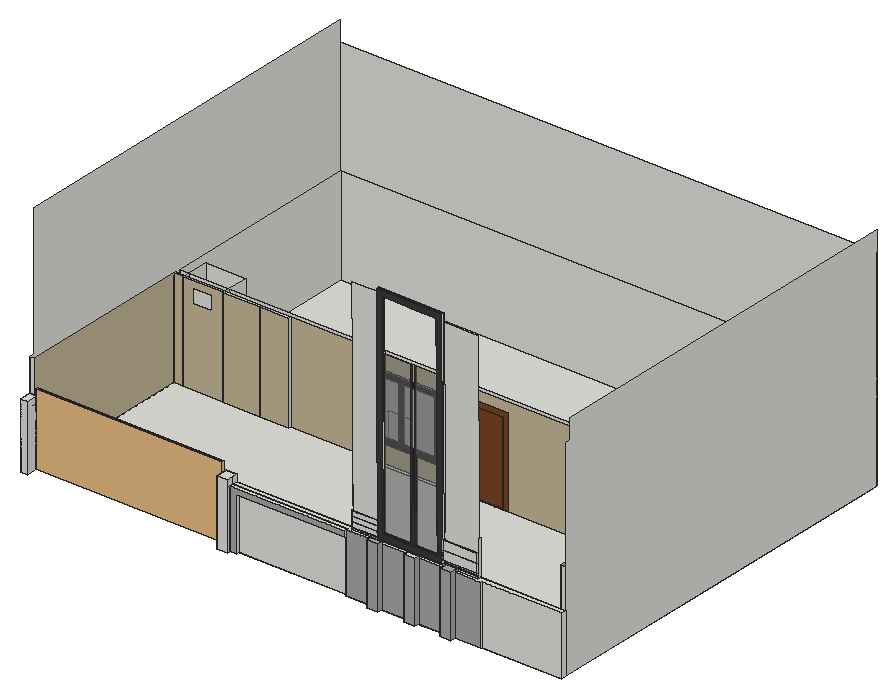
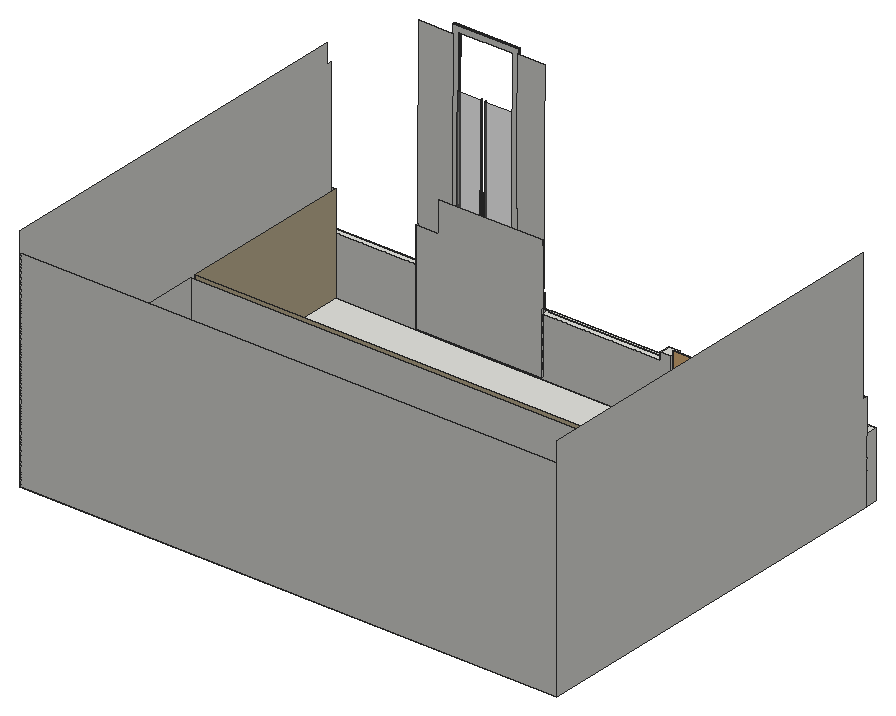
# SketchUp Ruby script. Lengths in inches.
U = 1.inch
M = Sketchup.active_model
def pt(a) = Geom::Point3d.new(a.map { |v| v * U })
def face(e, loops, mat)
  f = e.add_face(loops[0].map { |a| pt(a) })
  loops[1..].each { |l| e.add_face(l.map { |a| pt(a) }).erase! }
  f.material = f.back_material = mat if mat
  f
end
# faces: each face lists its corners as indices into pts; further lists are holes
def faces(e, pts, list, mat = nil) = list.each { |f| face(e, (f[0].is_a?(Array) ? f : [f]).map { |l| l.map { |i| pts[i] } }, mat) }
# xy, xz, yz: faces in a plane at the given z, y or x. An outline is a flat list of corners, or four numbers for a rectangle; further outlines are holes
def ring(l) = l.size == 4 ? [[l[0], l[1]], [l[2], l[1]], [l[2], l[3]], [l[0], l[3]]] : l.each_slice(2).to_a
def flat(e, list, mat, &to3) = list.each { |f| face(e, (f[0].is_a?(Array) ? f : [f]).map { |l| ring(l).map { |u, v| to3.(u, v) } }, mat) }
def xy(e, z, list, mat = nil) = flat(e, list, mat) { |x, y| [x, y, z] }
def xz(e, y, list, mat = nil) = flat(e, list, mat) { |x, z| [x, y, z] }
def yz(e, x, list, mat = nil) = flat(e, list, mat) { |y, z| [x, y, z] }
def lines(e, pts, list) = list.each { |a, b| e.add_line(pt(pts[a]), pt(pts[b])) }
# prism: a flat outline (further loops are holes) pulled along v
def prism(e, loops, v, mat = nil)
  f = face(e, loops, mat); d = Geom::Vector3d.new(v.map { |x| x * U })
  f.pushpull(f.normal.samedirection?(d) ? d.length : -d.length)
end
def box(e, o, s, mat = nil) = prism(e, [[o, [o[0] + s[0], o[1], o[2]], [o[0] + s[0], o[1] + s[1], o[2]], [o[0], o[1] + s[1], o[2]]]], [0, 0, s[2]], mat)
def at(x, y, z, deg = 0) = Geom::Transformation.translation(pt([x, y, z])) * Geom::Transformation.rotation(ORIGIN, Z_AXIS, deg.degrees)
def axes(o, x, y, z) = Geom::Transformation.new([*x, 0, *y, 0, *z, 0, *pt(o).to_a, 1])
def part(name) = M.definitions.add(name)
# library, detail: a bought-in or finely detailed component or shape, given as its bounding box
def library(name, o, s) = part(name).tap { |d| box(d.entities, o, s) }
def detail(e, o, s) = box(e.add_group.entities, o, s)
def put(e, d, t, mat = nil) = e.add_instance(d, t).tap { |i| i.material = mat if mat }
def group(e, t, mat = nil) = e.add_group.tap { |g| g.transformation = t; g.material = mat if mat }.entities
root = M.entities
M.materials.add("[0132_LightGray]").color = [169, 169, 169]
M.materials.add("[Color M07]").color = [58, 58, 58]
M.materials.add("[Color M08]").color = [30, 30, 30]
M.materials.add("[Quartz Light Brown]").color = [199, 184, 152]
M.materials.add("[Translucent Glass Gray]").color = [128, 128, 128]
M.materials["[Translucent Glass Gray]"].alpha = 0.5
M.materials.add("[Wood Veneer 01]").color = [120, 70, 37]
c1 = library("gate (1)",[0,0,0],[171.26,1.97,78.74])
prism(root,[[[595.0625,24.87,16.39],[825.84,24.87,16.39],[825.84,21.87,16.375],[595.0625,21.87,16.375]]],[0,-0.1,15.6875])
prism(root,[[[595.0625,24.87,36.02],[825.84,24.87,36.02],[825.84,21.74,36],[595.0625,21.74,36]]],[0,-0.1,15.6875])
prism(root,[[[595.0625,24.87,55.64],[825.84,24.87,55.64],[825.84,21.61,55.62],[595.0625,21.61,55.62]]],[0,-0.1,15.6875])
prism(root,[[[595.0625,24.87,75.27],[825.84,24.87,75.27],[825.84,21.48,75.25],[595.0625,21.48,75.25]]],[0,-0.1,15.6875])
xy(root,0,[[0,6,13.1875,18],[360,6,379.36,18],[634.43,6,654.87,15],[702.3,6,720,15],[720,6,722.74,15],
  [768.43,6,768.43,15,720,15,720,27,982.625,27,982.625,18,836.43,18,836.43,15,788.87,15,788.87,6],[379.36,12,391.35,18],[589.74,15,589.74,18,360,18,360,27,720,27,720,15],[0,18,13.1875,27],[0,27,0,738,982.625,738,982.625,729,9,729,9,359.125,25.58,359.125,25.58,350.125,9,350.125,9,27],
  [9,27,972.875,27,972.875,350.125,220.94,350.125,220.94,345.8125,99.55,345.8125,99.55,346.125,25.58,346.125,25.58,347.125,9,347.125],[972.875,27,972.875,350.125,608.23,350.125,608.23,353.125,514.29,353.125,514.29,350.125,439.49,350.125,439.49,352.625,397.49,352.625,397.49,350.125,99.55,350.125,99.55,359.125,982.625,359.125,982.625,27],[99.55,345.8125,167.26,350.125],[167.26,345.8125,220.94,350.125],[25.58,346.125,99.55,350.125],
  [9,347.125,25.58,350.125],[25.58,350.125,99.55,359.125],[397.49,350.125,400.49,352.625],[400.49,350.125,436.49,352.625],[436.49,350.125,439.49,352.625],
  [514.29,350.125,608.23,353.125],[9,359.125,25.58,359.125,25.58,398.125,99.55,398.125,99.55,359.125,972.875,359.125,972.875,729,9,729],[25.58,359.125,99.55,398.125],[972.875,359.125,982.625,729]])
xy(root,34.12,[[343.29,347.125,496.31,350.125]])
xy(root,43.35,[[419.8,347.125,426.4375,350.125]])
xy(root,43.35,[[352.52,347.125,419.8,350.125],[426.4375,347.125,487.09,350.125]],"[Color M08]")
xy(root,96.82,[[391.35,12,589.74,18]])
xy(root,108,[[379.36,6,379.39,12],[379.36,12,379.39,18],[379.39,12,589.74,18],[589.74,15,768.43,15,768.43,21.27,788.61,21.27,788.87,15,836.43,15,836.43,18,982.625,18,982.625,27,379.39,27,379.39,18,589.74,18]])
xy(root,111.5625,[[702.3,6,722.74,15]])
xy(root,111.5625,[[634.43,6,654.87,15],[768.43,6,788.87,6,788.87,15,788.61,21.27,768.43,21.27]],"[0132_LightGray]")
xy(root,112.12,[[595.0625,21.24,644.47,22.14]])
xy(root,120,[[0,6,13.1875,27],[360,6,379.36,6,379.36,18,379.39,18,379.39,27,360,27]])
xy(root,138.72,[[595.0625,21.07,644.47,22.09]])
xz(root,6,[[0,0,13.1875,120],[360,0,379.36,120]])
xz(root,6,[[634.43,0,654.87,111.5625],[702.3,0,722.74,111.5625],[768.43,0,788.87,111.5625]],"[0132_LightGray]")
xz(root,12,[[379.36,0,391.35,0,391.35,96.82,589.74,96.82,589.74,108,379.36,108]],"[0132_LightGray]")
xz(root,15,[[634.43,0,654.87,108],[702.3,0,722.74,108],[634.43,108,654.87,111.5625],[702.3,108,722.74,111.5625]])
xz(root,15,[[589.74,0,634.43,108],[654.87,0,702.3,108],[722.74,0,768.43,108],[788.87,0,836.43,108]],"[0132_LightGray]")
xz(root,18,[[379.36,0,379.36,108,589.74,108,589.74,96.82,391.35,96.82,391.35,0],[391.35,0,589.74,96.82],[836.43,0,982.625,108],[379.36,108,379.39,120]])
xz(root,21.27,[[768.43,108,788.61,111.5625]])
xz(root,27,[[0,0,9,108],[9,0,13.1875,108],[360,0,360,120,379.39,120,379.39,108,720,108,720,0],[720,0,972.875,108],[972.875,0,982.625,108],
  [0,108,9,120],[9,108,13.1875,120],[972.875,108,982.625,180],[0,120,9,180]])
xz(root,345.8125,[[99.55,0,167.26,180],[167.26,0,220.94,180]],"[Quartz Light Brown]")
xz(root,346.125,[[[25.58,0,99.55,180],[44.38,142.05,78.26,168.55]]],"[Quartz Light Brown]")
xz(root,347.125,[[[343.29,34.12,496.31,152.83],[352.52,43.35,487.09,143.6]],[419.8,43.35,426.4375,143.6]],"[Color M08]")
xz(root,347.125,[[9,0,25.58,180]],"[Quartz Light Brown]")
xz(root,350.125,[[9,0,25.58,180],[25.58,0,99.55,180],[99.55,0,167.26,180],[167.26,0,220.94,180],[[343.29,34.12,496.31,152.83],[352.52,43.35,487.09,143.6]],
  [419.8,43.35,426.4375,143.6]])
xz(root,350.125,[[[220.94,0,502.5625,0,502.5625,163.72,619.95,163.72,619.95,0,972.875,0,972.875,180,220.94,180],[343.29,34.12,496.31,152.83]]],"[Quartz Light Brown]")
xz(root,350.125,[[352.52,43.35,419.8,143.6],[426.4375,43.35,487.09,143.6]],"[Translucent Glass Gray]")
xz(root,350.125,[[502.5625,0,514.29,0,514.29,151.99,608.23,151.99,608.23,0,619.95,0,619.95,163.72,502.5625,163.72],[542.09,54.84,546.17,55.38,549.97,56.95,553.23,59.46,555.73,62.72,557.3,66.52,557.84,70.59,557.3,74.67,555.73,78.47,553.23,81.73,549.97,84.23,546.17,85.81,542.09,86.34,538.01,85.81,534.22,84.23,530.95,81.73,528.45,78.47,526.88,74.67,526.34,70.59,526.88,66.52,528.45,62.72,530.95,59.46,534.22,56.95,538.01,55.38]],"[Wood Veneer 01]")
xz(root,352.625,[[397.49,0,439.49,87]])
xz(root,353.125,[[542.09,54.84,538.01,55.38,534.22,56.95,530.95,59.46,528.45,62.72,526.88,66.52,526.34,70.59,526.88,74.67,528.45,78.47,530.95,81.73,534.22,84.23,538.01,85.81,542.09,86.34,546.17,85.81,549.97,84.23,553.23,81.73,555.73,78.47,557.3,74.67,557.84,70.59,557.3,66.52,555.73,62.72,553.23,59.46,549.97,56.95,546.17,55.38]])
xz(root,353.125,[[[514.29,0,608.23,151.99],[542.09,54.84,538.01,55.38,534.22,56.95,530.95,59.46,528.45,62.72,526.88,66.52,526.34,70.59,526.88,74.67,528.45,78.47,530.95,81.73,534.22,84.23,538.01,85.81,542.09,86.34,546.17,85.81,549.97,84.23,553.23,81.73,555.73,78.47,557.3,74.67,557.84,70.59,557.3,66.52,555.73,62.72,553.23,59.46,549.97,56.95,546.17,55.38]]],"[Wood Veneer 01]")
xz(root,359.125,[[9,0,972.875,180]])
xz(root,398.125,[[25.58,0,99.55,180]])
xz(root,729,[[9,0,972.875,180]])
xz(root,738,[[0,0,982.625,384]])
yz(root,0,[[6,0,27,120],[27,0,27,180,36,180,36,420,738,420,738,0]])
yz(root,9,[[347.125,0,350.125,180],[359.125,0,729,180]])
yz(root,9,[[27,0,347.125,180]],"[Quartz Light Brown]")
yz(root,13.1875,[[6,0,27,120]])
yz(root,25.58,[[346.125,0,347.125,180],[347.125,0,350.125,180],[350.125,0,398.125,180]])
yz(root,99.55,[[345.8125,0,346.125,180],[346.125,0,350.125,180],[350.125,0,398.125,180]])
yz(root,167.26,[[345.8125,0,350.125,180]])
yz(root,220.94,[[345.8125,0,350.125,180]])
yz(root,343.29,[[347.125,34.12,350.125,152.83]],"[Color M08]")
yz(root,352.52,[[347.125,43.35,350.125,143.6]],"[Color M08]")
yz(root,360,[[6,0,27,120]])
yz(root,379.36,[[6,0,12,108],[12,0,18,108],[6,108,18,120]])
yz(root,379.39,[[18,108,27,120]])
yz(root,391.35,[[12,0,18,96.82]])
yz(root,419.8,[[347.125,43.35,350.125,143.6]],"[Color M08]")
yz(root,426.4375,[[347.125,43.35,350.125,143.6]],"[Color M08]")
yz(root,487.09,[[347.125,43.35,350.125,143.6]],"[Color M08]")
yz(root,496.31,[[347.125,34.12,350.125,152.83]],"[Color M08]")
yz(root,514.29,[[350.125,0,353.125,151.99]],"[Wood Veneer 01]")
yz(root,589.74,[[15,0,18,96.82],[12,96.82,15,108],[15,96.82,18,108]])
yz(root,595.0625,[[25.47,2.61,24.87,94.89,24.76,110.58,24.3125,180,27,180,27,227.94,28.47,2.63],[21.36,94.87,21.25,110.56,24.76,110.58,24.87,94.89],[21.24,112.12,21.19,120.34,22.09,120.35,22.14,112.12],[21.18,121.3,21.13,129.53,22.09,129.54,22.14,121.31],[21.125,130.49,21.07,138.72,22.09,138.72,22.14,130.5]])
yz(root,608.23,[[350.125,0,353.125,151.99]],"[Wood Veneer 01]")
yz(root,634.43,[[6,0,15,111.5625]],"[0132_LightGray]")
yz(root,644.47,[[21.76,111.28,21.75,112.12,22.14,112.12,24.75,112.14,24.76,111.3],[21.24,112.12,21.19,120.34,21.7,120.35,21.75,112.12],[21.75,112.12,21.7,120.35,22.09,120.35,22.14,112.12],[22.14,112.12,22.09,120.35,24.7,120.37,24.75,112.14],[21.7,120.35,21.69,121.31,22.14,121.31,24.69,121.33,24.7,120.37,22.09,120.35],
  [21.18,121.3,21.13,129.53,21.64,129.53,21.69,121.31],[21.69,121.31,21.64,129.53,22.09,129.54,22.14,121.31],[22.14,121.31,22.09,129.54,24.64,129.55,24.69,121.33],[21.64,129.53,21.63,130.49,22.14,130.5,24.63,130.51,24.64,129.55,22.09,129.54],[21.125,130.49,21.07,138.72,21.58,138.72,21.63,130.49],
  [21.63,130.49,21.58,138.72,22.09,138.72,22.14,130.5],[22.14,130.5,22.09,138.72,24.58,138.74,24.63,130.51],[21.58,138.72,21.57,139.68,22.14,139.68,24.57,139.7,24.58,138.74,22.09,138.72]])
yz(root,644.47,[[18.76,111.26,18.75,112.1,21.24,112.12,21.75,112.12,21.76,111.28],[18.75,112.1,18.7,120.33,21.19,120.34,21.24,112.12],[18.7,120.33,18.69,121.29,21.18,121.3,21.69,121.31,21.7,120.35,21.19,120.34],[18.69,121.29,18.64,129.51,21.13,129.53,21.18,121.3],[18.64,129.51,18.63,130.47,21.125,130.49,21.63,130.49,21.64,129.53,21.13,129.53],
  [18.63,130.47,18.58,138.7,21.07,138.72,21.125,130.49],[18.58,138.7,18.57,139.66,21.0625,139.68,21.57,139.68,21.58,138.72,21.07,138.72]],"[Color M07]")
yz(root,653.47,[[18.7,120.26,21.7,120.28,21.26,187.5,18.26,187.48],[21.7,120.28,24.7,120.3,24.26,187.52,22.78,187.51,21.26,187.5]],"[Color M07]")
yz(root,654.87,[[6,0,15,111.5625]],"[0132_LightGray]")
yz(root,702.3,[[6,0,15,111.5625]],"[0132_LightGray]")
yz(root,703.69,[[21.7,120.28,21.26,187.5,21.22,194.61,20.77,263.62,20.72,270.73,20.27,339.74,20.23,346.86,19.78,415.86,22.78,415.88,24.7,120.3]],"[Color M07]")
yz(root,710.84,[[21.7,120.28,24.7,120.3,22.78,415.88,19.78,415.86,20.23,346.86,20.27,339.74,20.72,270.73,20.77,263.62,21.22,194.61,21.26,187.5]],"[Color M07]")
yz(root,722.74,[[6,0,15,111.5625]],"[0132_LightGray]")
yz(root,753.91,[[18.7,120.26,18.26,187.48,21.26,187.5,21.7,120.28],[21.7,120.28,21.26,187.5,22.78,187.51,24.26,187.52,24.7,120.3]],"[Color M07]")
yz(root,762.91,[[18.76,111.26,21.76,111.28,21.72,117.24,20.16,117.23,18.72,117.23],[21.76,111.28,24.76,111.3,24.72,117.26,22.1875,117.25,21.72,117.24],[18.72,117.23,20.16,117.23,20.06,132.84,18.62,132.83],[20.16,117.23,21.72,117.24,21.62,132.85,20.06,132.84],[21.72,117.24,22.1875,117.25,22.09,132.85,21.62,132.85],
  [22.1875,117.25,24.72,117.26,24.62,132.87,22.09,132.85],[18.62,132.83,20.06,132.84,21.62,132.85,21.61,133.99,20.05,133.98,18.61,133.97],[21.62,132.85,22.09,132.85,24.62,132.87,24.61,134.01,22.1875,134,21.61,133.99],[18.61,133.97,20.05,133.98,19.95,149.59,18.51,149.58],[20.05,133.98,21.61,133.99,21.51,149.6,19.95,149.59],
  [21.61,133.99,22.1875,134,22.09,149.6,21.51,149.6],[22.1875,134,24.61,134.01,24.51,149.61,22.09,149.6]])
yz(root,768.43,[[6,0,6,111.5625,21.27,111.5625,21.27,108,15,108,15,0]],"[0132_LightGray]")
yz(root,788.87,[[6,0,15,111.5625]],"[0132_LightGray]")
yz(root,825.84,[[25.47,2.61,28.47,2.63,27.36,172.4375,24.36,172.42,24.76,110.58,24.87,94.89],[21.36,94.87,24.87,94.89,24.76,110.58,21.25,110.56],[20.16,117.23,22.1875,117.25,22.09,132.85,20.06,132.84],[20.05,133.98,22.1875,134,22.09,149.6,19.95,149.59]])
yz(root,836.43,[[15,0,18,108]])
yz(root,972.875,[[359.125,0,729,180]])
yz(root,972.875,[[27,0,350.125,180]],"[Quartz Light Brown]")
yz(root,982.625,[[18,0,27,108],[27,0,738,0,738,420,35.0625,420,35.0625,384,27,384]])
p = [[825.84,25.47,2.61],[825.84,24.87,94.89],[595.0625,24.87,94.89],[595.0625,25.47,2.61],[595.0625,28.47,2.63],[825.84,28.47,2.63],
  [595.0625,27,227.94],[784.34,27,227.94],[784.34,27.36,172.4375],[825.84,27.36,172.4375],[538.01,353.125,55.38],[542.09,353.125,54.84],
  [542.09,350.125,54.84],[538.01,350.125,55.38],[546.17,353.125,55.38],[546.17,350.125,55.38],[534.22,353.125,56.95],[534.22,350.125,56.95],
  [549.97,353.125,56.95],[549.97,350.125,56.95],[530.95,353.125,59.46],[530.95,350.125,59.46],[553.23,353.125,59.46],[553.23,350.125,59.46],
  [528.45,353.125,62.72],[528.45,350.125,62.72],[555.73,353.125,62.72],[555.73,350.125,62.72],[526.88,353.125,66.52],[526.88,350.125,66.52],
  [557.3,353.125,66.52],[557.3,350.125,66.52],[526.34,353.125,70.59],[526.34,350.125,70.59],[557.84,353.125,70.59],[557.84,350.125,70.59],
  [526.88,353.125,74.67],[526.88,350.125,74.67],[557.3,353.125,74.67],[557.3,350.125,74.67],[528.45,353.125,78.47],[528.45,350.125,78.47],
  [555.73,353.125,78.47],[555.73,350.125,78.47],[530.95,353.125,81.73],[530.95,350.125,81.73],[553.23,353.125,81.73],[553.23,350.125,81.73],
  [534.22,353.125,84.23],[534.22,350.125,84.23],[549.97,353.125,84.23],[549.97,350.125,84.23],[538.01,353.125,85.81],[538.01,350.125,85.81],
  [546.17,353.125,85.81],[546.17,350.125,85.81],[542.09,353.125,86.34],[542.09,350.125,86.34],[595.0625,21.25,110.56],[595.0625,21.36,94.87],
  [825.84,21.36,94.87],[825.84,21.25,110.56],[595.0625,24.76,110.58],[825.84,24.76,110.58],[788.87,15,108],[788.61,21.27,108],
  [788.61,21.27,111.5625],[788.87,15,111.5625],[595.0625,24.3125,180],[825.84,24.36,172.42],[825.84,24.28,184.45],[825.84,24.18,200.05],
  [825.84,24,227.98],[825.84,22.1875,506.25],[762.91,22.1875,506.25],[762.91,23.52,301.67],[762.91,23.62,286.07],[762.91,23.63,284.73],
  [762.91,23.73,269.13],[762.91,23.74,267.8],[762.91,23.84,252.2],[762.91,23.85,250.86],[762.91,23.95,235.26],[762.91,23.96,233.92],
  [762.91,24.0625,218.32],[762.91,24.07,216.99],[762.91,24.17,201.39],[762.91,24.18,200.05],[762.91,24.28,184.45],[762.91,24.29,183.11],
  [762.91,24.39,167.51],[762.91,24.4,166.36],[762.91,24.5,150.76],[762.91,24.51,149.61],[762.91,24.61,134.01],[762.91,24.62,132.87],
  [762.91,24.72,117.26],[762.91,24.76,111.3],[644.47,24.76,111.3],[644.47,24.75,112.14],[644.47,24.7,120.37],[644.47,24.69,121.33],
  [644.47,24.64,129.55],[644.47,24.63,130.51],[644.47,24.58,138.74],[644.47,24.57,139.7],[644.47,24.52,147.93],[644.47,24.52,148.89],
  [644.47,24.46,157.11],[644.47,24.46,158.07],[644.47,24.4,166.3],[644.47,24.4,167.26],[644.47,24.34,175.49],[644.47,24.34,176.45],
  [644.47,24.28,184.68],[644.47,24.28,185.64],[644.47,24.22,193.86],[644.47,24.22,194.82],[644.47,24.16,203.05],[644.47,24.16,204.01],
  [644.47,24.1,212.24],[644.47,24.1,213.2],[644.47,24.04,221.42],[644.47,24.04,222.38],[644.47,23.98,230.61],[644.47,23.98,231.57],
  [644.47,23.92,239.8],[644.47,23.92,240.76],[644.47,23.86,248.99],[644.47,23.86,249.95],[644.47,23.8,258.17],[644.47,23.8,259.13],
  [644.47,23.74,267.36],[644.47,23.74,268.32],[644.47,23.68,276.55],[644.47,23.67,278.13],[644.47,23.62,286.36],[644.47,23.61,287.94],
  [644.47,23.56,296.17],[644.47,23.55,297.76],[644.47,23.49,305.98],[644.47,23.48,307.57],[644.47,23.43,315.8],[644.47,23.42,317.38],
  [644.47,23.36,325.61],[644.47,23.35,327.19],[644.47,23.3,335.42],[644.47,23.29,337],[644.47,23.24,345.23],[644.47,23.23,346.82],
  [644.47,23.17,355.04],[644.47,23.16,356.63],[644.47,23.11,364.86],[644.47,23.1,366.44],[644.47,23.04,374.67],[644.47,23.03,376.25],
  [644.47,22.98,384.48],[644.47,22.97,386.0625],[644.47,22.92,394.29],[644.47,22.91,395.875],[644.47,22.85,404.1],[644.47,22.84,405.6875],
  [644.47,22.79,413.92],[644.47,22.78,415.5],[644.47,22.73,423.73],[644.47,22.72,425.3125],[644.47,22.66,433.54],[644.47,22.65,435.125],
  [644.47,22.6,443.35],[644.47,22.59,444.9375],[644.47,22.53,453.16],[644.47,22.52,454.75],[644.47,22.47,462.98],[644.47,22.46,464.5625],
  [644.47,22.41,472.79],[644.47,22.4,474.375],[644.47,22.34,482.6],[644.47,22.33,484.19],[644.47,22.28,492.41],[644.47,22.27,494],
  [644.47,22.21,502.22],[644.47,22.2,503.81],[644.47,22.15,512.04],[644.47,22.14,513.62],[595.0625,22.14,513.62],[595.0625,22.92,393.5625],
  [595.0625,23.0625,371.92],[595.0625,24,227.98],[644.47,18.76,111.26],[762.91,18.76,111.26],[762.91,18.72,117.23],[762.91,18.62,132.83],
  [762.91,18.61,133.97],[762.91,18.51,149.58],[762.91,18.5,150.72],[762.91,18.4,166.33],[762.91,18.39,167.47],[762.91,18.29,183.07],
  [762.91,18.28,184.41],[762.91,18.18,200.01],[762.91,18.17,201.35],[762.91,18.07,216.95],[762.91,18.0625,218.28],[762.91,17.96,233.88],
  [762.91,17.95,235.22],[762.91,17.85,250.82],[762.91,17.84,252.16],[762.91,17.74,267.76],[762.91,17.73,269.09],[762.91,17.63,284.7],
  [762.91,17.62,286.03],[762.91,17.52,301.63],[762.91,16.09,521.81],[644.47,16.09,521.81],[644.47,16.14,513.58],[644.47,16.15,512],
  [644.47,16.2,503.77],[644.47,16.21,502.1875],[644.47,16.27,493.96],[644.47,16.28,492.375],[644.47,16.33,484.15],[644.47,16.34,482.5625],
  [644.47,16.4,474.33],[644.47,16.41,472.75],[644.47,16.46,464.52],[644.47,16.47,462.9375],[644.47,16.52,454.71],[644.47,16.53,453.125],
  [644.47,16.59,444.9],[644.47,16.6,443.3125],[644.47,16.65,435.09],[644.47,16.66,433.5],[644.47,16.72,425.27],[644.47,16.73,423.6875],
  [644.47,16.78,415.46],[644.47,16.79,413.88],[644.47,16.84,405.65],[644.47,16.85,404.07],[644.47,16.91,395.84],[644.47,16.92,394.25],
  [644.47,16.97,386.03],[644.47,16.98,384.44],[644.47,17.03,376.21],[644.47,17.05,374.63],[644.47,17.1,366.4],[644.47,17.11,364.82],
  [644.47,17.16,356.59],[644.47,17.17,355],[644.47,17.23,346.78],[644.47,17.24,345.19],[644.47,17.29,336.96],[644.47,17.3,335.38],
  [644.47,17.35,327.15],[644.47,17.36,325.57],[644.47,17.42,317.34],[644.47,17.43,315.76],[644.47,17.48,307.53],[644.47,17.49,305.94],
  [644.47,17.55,297.72],[644.47,17.56,296.13],[644.47,17.61,287.9],[644.47,17.62,286.32],[644.47,17.67,278.09],[644.47,17.68,276.51],
  [644.47,17.74,268.28],[644.47,17.74,267.32],[644.47,17.8,259.09],[644.47,17.8,258.13],[644.47,17.86,249.91],[644.47,17.86,248.95],
  [644.47,17.92,240.72],[644.47,17.92,239.76],[644.47,17.98,231.53],[644.47,17.98,230.57],[644.47,18.04,222.34],[644.47,18.04,221.39],
  [644.47,18.1,213.16],[644.47,18.1,212.2],[644.47,18.16,203.97],[644.47,18.16,203.01],[644.47,18.22,194.78],[644.47,18.22,193.82],
  [644.47,18.28,185.6],[644.47,18.28,184.64],[644.47,18.34,176.41],[644.47,18.34,175.45],[644.47,18.4,167.22],[644.47,18.4,166.26],
  [644.47,18.46,158.03],[644.47,18.46,157.08],[644.47,18.52,148.85],[644.47,18.52,147.89],[644.47,18.57,139.66],[644.47,18.58,138.7],
  [644.47,18.63,130.47],[644.47,18.64,129.51],[644.47,18.69,121.29],[644.47,18.7,120.33],[644.47,18.75,112.1],[753.91,16.15,512.81],
  [753.91,16.73,422.96],[753.91,16.78,415.84],[753.91,17.23,346.84],[753.91,17.27,339.72],[753.91,17.72,270.71],[753.91,17.77,263.6],
  [753.91,18.22,194.59],[753.91,18.26,187.48],[753.91,18.7,120.26],[710.84,18.7,120.26],[703.69,18.7,120.26],[653.47,18.7,120.26],
  [653.47,18.26,187.48],[653.47,18.22,194.59],[653.47,17.77,263.6],[653.47,17.72,270.71],[653.47,17.27,339.72],[653.47,17.23,346.84],
  [653.47,16.78,415.84],[653.47,16.73,422.96],[653.47,16.15,512.81],[703.69,16.15,512.81],[710.84,16.15,512.81],[644.47,21.76,111.28],
  [762.91,21.76,111.28],[644.47,21.75,112.12],[644.47,21.7,120.35],[644.47,21.69,121.31],[644.47,21.64,129.53],[644.47,21.63,130.49],
  [644.47,21.58,138.72],[644.47,21.57,139.68],[644.47,21.52,147.91],[644.47,21.52,148.87],[644.47,21.46,157.1],[644.47,21.46,158.05],
  [644.47,21.4,166.28],[644.47,21.4,167.24],[644.47,21.34,175.47],[644.47,21.34,176.43],[644.47,21.28,184.66],[644.47,21.28,185.62],
  [644.47,21.22,193.84],[644.47,21.22,194.8],[644.47,21.16,203.03],[644.47,21.16,203.99],[644.47,21.1,212.22],[644.47,21.1,213.18],
  [644.47,21.04,221.4],[644.47,21.04,222.36],[644.47,20.98,230.59],[644.47,20.98,231.55],[644.47,20.92,239.78],[644.47,20.92,240.74],
  [644.47,20.86,248.97],[644.47,20.86,249.93],[644.47,20.8,258.15],[644.47,20.8,259.11],[644.47,20.74,267.34],[644.47,20.74,268.3],
  [644.47,20.68,276.53],[644.47,20.67,278.11],[644.47,20.62,286.34],[644.47,20.61,287.92],[644.47,20.56,296.15],[644.47,20.55,297.74],
  [644.47,20.49,305.96],[644.47,20.48,307.55],[644.47,20.43,315.78],[644.47,20.42,317.36],[644.47,20.36,325.59],[644.47,20.35,327.17],
  [644.47,20.3,335.4],[644.47,20.29,336.98],[644.47,20.24,345.21],[644.47,20.23,346.8],[644.47,20.17,355.02],[644.47,20.16,356.61],
  [644.47,20.11,364.84],[644.47,20.1,366.42],[644.47,20.04,374.65],[644.47,20.03,376.23],[644.47,19.98,384.46],[644.47,19.97,386.04],
  [644.47,19.92,394.27],[644.47,19.91,395.86],[644.47,19.85,404.08],[644.47,19.84,405.67],[644.47,19.79,413.9],[644.47,19.78,415.48],
  [644.47,19.73,423.71],[644.47,19.72,425.29],[644.47,19.66,433.52],[644.47,19.65,435.11],[644.47,19.6,443.33],[644.47,19.59,444.92],
  [644.47,19.53,453.14],[644.47,19.52,454.73],[644.47,19.47,462.96],[644.47,19.46,464.54],[644.47,19.41,472.77],[644.47,19.4,474.35],
  [644.47,19.34,482.58],[644.47,19.33,484.17],[644.47,19.28,492.39],[644.47,19.27,493.98],[644.47,19.21,502.21],[644.47,19.2,503.79],
  [644.47,19.15,512.02],[644.47,19.14,513.6],[644.47,19.09,521.83],[762.91,19.09,521.83],[762.91,20.52,301.65],[762.91,20.62,286.05],
  [762.91,20.63,284.71],[762.91,20.73,269.11],[762.91,20.74,267.78],[762.91,20.84,252.18],[762.91,20.85,250.84],[762.91,20.95,235.24],
  [762.91,20.96,233.9],[762.91,21.0625,218.3],[762.91,21.07,216.97],[762.91,21.17,201.37],[762.91,21.18,200.03],[762.91,21.28,184.43],
  [762.91,21.29,183.09],[762.91,21.39,167.49],[762.91,21.4,166.34],[762.91,21.5,150.74],[762.91,21.51,149.6],[762.91,21.61,133.99],
  [762.91,21.62,132.85],[762.91,21.72,117.24],[753.91,19.73,422.98],[753.91,19.15,512.83],[710.84,19.15,512.83],[703.69,19.15,512.83],
  [653.47,19.15,512.83],[653.47,19.73,422.98],[653.47,19.78,415.86],[653.47,20.23,346.86],[653.47,20.27,339.74],[653.47,20.72,270.73],
  [653.47,20.77,263.62],[653.47,21.22,194.61],[653.47,21.26,187.5],[653.47,21.7,120.28],[703.69,21.7,120.28],[710.84,21.7,120.28],
  [753.91,21.7,120.28],[753.91,21.26,187.5],[753.91,21.22,194.61],[753.91,20.77,263.62],[753.91,20.72,270.73],[753.91,20.27,339.74],
  [753.91,20.23,346.86],[753.91,19.78,415.86],[644.47,22.09,521.85],[762.91,22.09,521.85],[753.91,22.73,423],[753.91,22.15,512.85],
  [710.84,22.15,512.85],[703.69,22.15,512.85],[653.47,22.15,512.85],[653.47,22.73,423],[653.47,22.78,415.88],[653.47,23.23,346.875],
  [653.47,23.27,339.76],[653.47,23.72,270.75],[653.47,23.77,263.64],[653.47,24.22,194.63],[653.47,24.26,187.52],[653.47,24.7,120.3],
  [703.69,24.7,120.3],[710.84,24.7,120.3],[753.91,24.7,120.3],[753.91,24.26,187.52],[753.91,24.22,194.63],[753.91,23.77,263.64],
  [753.91,23.72,270.75],[753.91,23.27,339.76],[753.91,23.23,346.875],[753.91,22.78,415.88],[595.0625,21.19,120.34],[595.0625,21.24,112.12],
  [644.47,21.24,112.12],[644.47,21.19,120.34],[595.0625,22.14,112.12],[595.0625,22.09,120.35],[644.47,22.09,120.35],[644.47,22.14,112.12],
  [762.91,20.06,132.84],[762.91,20.16,117.23],[825.84,20.16,117.23],[825.84,20.06,132.84],[762.91,22.1875,117.25],[825.84,22.1875,117.25],
  [762.91,22.09,132.85],[825.84,22.09,132.85],[710.84,21.26,187.5],[703.69,21.26,187.5],[703.69,22.78,415.88],[710.84,22.78,415.88],
  [595.0625,21.13,129.53],[595.0625,21.18,121.3],[644.47,21.18,121.3],[644.47,21.13,129.53],[595.0625,22.14,121.31],[644.47,22.14,121.31],
  [595.0625,22.09,129.54],[644.47,22.09,129.54],[595.0625,21.07,138.72],[595.0625,21.125,130.49],[644.47,21.125,130.49],[644.47,21.07,138.72],
  [595.0625,22.14,130.5],[644.47,22.14,130.5],[595.0625,22.09,138.72],[644.47,22.09,138.72],[762.91,19.95,149.59],[762.91,20.05,133.98],
  [825.84,20.05,133.98],[825.84,19.95,149.59],[762.91,22.1875,134],[825.84,22.1875,134],[762.91,22.09,149.6],[825.84,22.09,149.6],
  [825.84,24.76,12.46],[595.0625,24.76,12.46],[13.1875,18,108],[13.1875,27,108],[397.49,350.125,87],[397.49,352.625,87],
  [439.49,350.125,87],[439.49,352.625,87]]
faces(root,p,[[0,1,2,3],[4,5,0,3],[4,6,7,8,9,5],[58,59,60,61],[2,1,60,59],[2,62,63,1],[63,62,58,61],[68,62,63,69,70,71,72,73,74,75,76,77,78,79,80,81,82,83,84,85,86,87,88,89,90,91,92,93,94,95,96,97,98,99,100,101,102,103,104,105,106,107,108,109,110,111,112,113,114,115,116,117,118,119,120,121,122,123,124,125,126,127,128,129,130,131,132,133,134,135,136,137,138,139,140,141,142,143,144,145,146,147,148,149,150,151,152,153,154,155,156,157,158,159,160,161,162,163,164,165,166,167,168,169,170,171,172,173,174,175,176,177,178,179,180,181,182,183,184,185,186,187],
  [[324,323,325,326,327,328,329,330,331,332,333,334,335,336,337,338,339,340,341,342,343,344,345,346,347,348,349,350,351,352,353,354,355,356,357,358,359,360,361,362,363,364,365,366,367,368,369,370,371,372,373,374,375,376,377,378,379,380,381,382,383,384,385,386,387,388,389,390,391,392,393,394,395,396,397,398,399,400,401,402,403,404,405,406,407,408,409,410,411,412,413,414,415,416,417,418,419,420,421,422,423,424,425,426,427,428,429,430,431,432,433],[434,435,436,437,438,439,440,441,442,443,444,445,446,447,448,449,450,451,452,453,454,455,456,457]],[[97,98,99,100,101,102,103,104,105,106,107,108,109,110,111,112,113,114,115,116,117,118,119,120,121,122,123,124,125,126,127,128,129,130,131,132,133,134,135,136,137,138,139,140,141,142,143,144,145,146,147,148,149,150,151,152,153,154,155,156,157,158,159,160,161,162,163,164,165,166,167,168,169,170,171,172,173,174,175,176,177,178,179,180,181,182,183,458,459,74,75,76,77,78,79,80,81,82,83,84,85,86,87,88,89,90,91,92,93,94,95,96],[460,461,462,463,464,465,466,467,468,469,470,471,472,473,474,475,476,477,478,479,480,481,482,483]],[484,485,486,487],[488,489,490,491],[492,493,494,495],[496,497,494,493,433],[496,498,499,497],[490,489,484,487,326],
  [448,449,475,474],[504,505,506,507],[508,509,327,506,505],[508,510,511,509],[511,510,504,507,328],[512,513,514,515],[516,517,329,514,513],[516,518,519,517],
  [499,498,432,492,495],[520,521,522,523],[524,525,522,521,431],[524,526,527,525]])
faces(root,p,[[10,11,12,13],[11,14,15,12],[16,10,13,17],[14,18,19,15],[20,16,17,21],[18,22,23,19],[24,20,21,25],[22,26,27,23],
  [28,24,25,29],[26,30,31,27],[32,28,29,33],[30,34,35,31],[36,32,33,37],[34,38,39,35],[40,36,37,41],[38,42,43,39],
  [44,40,41,45],[42,46,47,43],[48,44,45,49],[46,50,51,47],[52,48,49,53],[50,54,55,51],[56,52,53,57],[54,56,57,55]],"[Wood Veneer 01]")
faces(root,p,[[64,65,66,67]],"[0132_LightGray]")
faces(root,p,[[[188,189,190,191,192,193,194,195,196,197,198,199,200,201,202,203,204,205,206,207,208,209,210,211,212,213,214,215,216,217,218,219,220,221,222,223,224,225,226,227,228,229,230,231,232,233,234,235,236,237,238,239,240,241,242,243,244,245,246,247,248,249,250,251,252,253,254,255,256,257,258,259,260,261,262,263,264,265,266,267,268,269,270,271,272,273,274,275,276,277,278,279,280,281,282,283,284,285,286,287,288,289,290,291,292,293,294,295,296,297,298],[299,300,301,302,303,304,305,306,307,308,309,310,311,312,313,314,315,316,317,318,319,320,321,322]],[323,324,189,188],[98,97,324,323],[448,447,311,310],[449,448,310,309],[450,449,309,308],[449,500,501,448],[474,473,447,448],
  [476,475,449,450]],"[Color M07]")
faces(root,p,[[474,502,466,467,468,469,470,471,472,473],[482,483,503,475,476,477,478,479,480,481]],"[Translucent Glass Gray]")
lines(root,p,[[528,529],[530,531],[532,533],[534,535]])
put(root,c1,axes([13.1875,25.68,0],[1.9873,0,0],[0,1.67,0],[0,0,1.67]))
